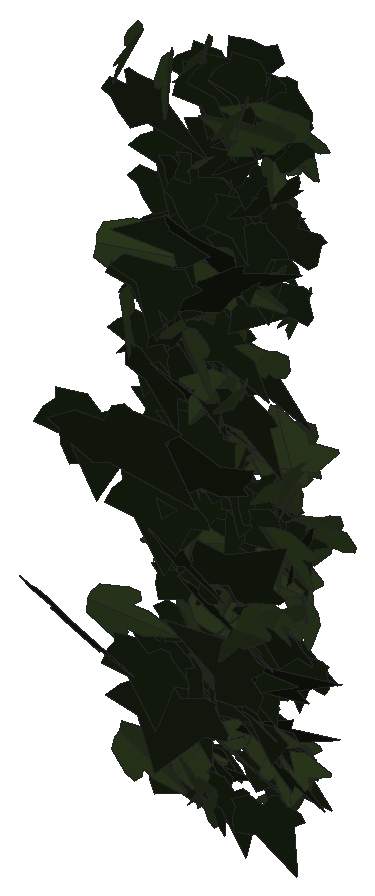
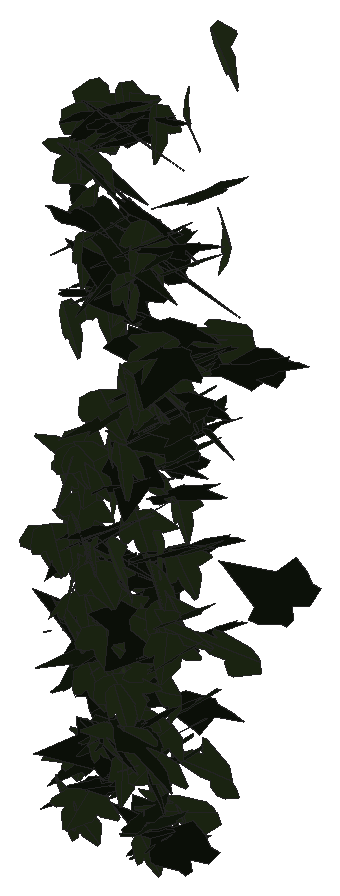
# SketchUp Ruby script. Lengths in millimetres.
U = 1.mm
M = Sketchup.active_model
def pt(a) = Geom::Point3d.new(a.map { |v| v * U })
def face(e, loops, mat)
  f = e.add_face(loops[0].map { |a| pt(a) })
  loops[1..].each { |l| e.add_face(l.map { |a| pt(a) }).erase! }
  f.material = f.back_material = mat if mat
  f
end
# faces: each face lists its corners as indices into pts; further lists are holes
def faces(e, pts, list, mat = nil) = list.each { |f| face(e, (f[0].is_a?(Array) ? f : [f]).map { |l| l.map { |i| pts[i] } }, mat) }
# xy, xz, yz: faces in a plane at the given z, y or x. An outline is a flat list of corners, or four numbers for a rectangle; further outlines are holes
def ring(l) = l.size == 4 ? [[l[0], l[1]], [l[2], l[1]], [l[2], l[3]], [l[0], l[3]]] : l.each_slice(2).to_a
def flat(e, list, mat, &to3) = list.each { |f| face(e, (f[0].is_a?(Array) ? f : [f]).map { |l| ring(l).map { |u, v| to3.(u, v) } }, mat) }
def xy(e, z, list, mat = nil) = flat(e, list, mat) { |x, y| [x, y, z] }
def xz(e, y, list, mat = nil) = flat(e, list, mat) { |x, z| [x, y, z] }
def yz(e, x, list, mat = nil) = flat(e, list, mat) { |y, z| [x, y, z] }
def lines(e, pts, list) = list.each { |a, b| e.add_line(pt(pts[a]), pt(pts[b])) }
# prism: a flat outline (further loops are holes) pulled along v
def prism(e, loops, v, mat = nil)
  f = face(e, loops, mat); d = Geom::Vector3d.new(v.map { |x| x * U })
  f.pushpull(f.normal.samedirection?(d) ? d.length : -d.length)
end
def box(e, o, s, mat = nil) = prism(e, [[o, [o[0] + s[0], o[1], o[2]], [o[0] + s[0], o[1] + s[1], o[2]], [o[0], o[1] + s[1], o[2]]]], [0, 0, s[2]], mat)
def at(x, y, z, deg = 0) = Geom::Transformation.translation(pt([x, y, z])) * Geom::Transformation.rotation(ORIGIN, Z_AXIS, deg.degrees)
def axes(o, x, y, z) = Geom::Transformation.new([*x, 0, *y, 0, *z, 0, *pt(o).to_a, 1])
def part(name) = M.definitions.add(name)
# library, detail: a bought-in or finely detailed component or shape, given as its bounding box
def library(name, o, s) = part(name).tap { |d| box(d.entities, o, s) }
def detail(e, o, s) = box(e.add_group.entities, o, s)
def put(e, d, t, mat = nil) = e.add_instance(d, t).tap { |i| i.material = mat if mat }
def group(e, t, mat = nil) = e.add_group.tap { |g| g.transformation = t; g.material = mat if mat }.entities
root = M.entities
M.materials.add("efeu1").color = [18, 25, 13]
M.materials.add("efeu2").color = [43, 57, 29]
c1 = part("ivyleaf_10")
p = [[0,12.8,-0.8],[-1.5,51.3,-10.9],[-4.9,51,-11.6],[-13.6,26.5,-7.3],[-13.2,15.9,-4.6],[-21.1,19.3,-7.2],
  [-29.5,16.3,-8.3],[-29.2,8.3,-6.2],[-19.7,-9.8,0.5],[-7.6,-13,4],[1,-12.2,5.8],[-0.4,51.1,-11.1],
  [-1.5,51.1,-10.9],[1,-12.4,5.9],[16.9,-12.4,3.5],[35.1,9.1,-5.1],[35,12.9,-6.1],[20.5,16.4,-4.9],
  [15.8,15,-3.8],[15.3,27.6,-7.1],[12.8,31.3,-7.8]]
faces(c1.entities,p,[[0,1,2,3,4,5,6,7,8,9,10],[11,12,0,13,14,15,16,17,18,19,20]],"efeu2")
c2 = part("ivyleaf_9")
p = [[39.1,54.8,31.7],[34.5,51.8,30.2],[-5.3,25.2,17.3],[-17.9,28.3,20.9],[-21.6,21.7,17],[-20.2,4.3,5.3],
  [-22.9,-0.3,2.5],[-17.1,-4,-0.6],[-2,-2.1,-1.2],[-0.7,-15.4,-10.1],[16.6,-22.3,-16.7],[21.1,-15.1,-12.5],
  [32.7,-10.7,-11],[46.1,-1.8,-6.6],[30.8,11.2,3.8]]
faces(c2.entities,p,[[0,1,2,3,4,5,6,7,8,9,10,11,12,13,14]],"efeu1")
put(root,c1,axes([1806.8,852.7,2286.1],[-0.01789,-0.27296,-1.00474],[1.7176,0.4989,-0.14398],[0.98809,-0.87218,0.23209]))
put(root,c2,axes([1814.5,923.6,2199.2],[0.8191,-0.82834,0.03911],[0.07035,-0.02486,-0.93323],[1.57668,0.43144,0.02132]))
put(root,c2,axes([1832.8,891.2,2170.1],[-0.57727,-0.84907,0.25897],[-0.09922,-0.25616,-0.90092],[1.68653,-0.30569,0.03564]))
put(root,c1,axes([1839.7,935.9,1905.6],[-0.70225,-0.77074,-0.26118],[0.21308,0.23596,-0.85451],[1.53408,-0.38559,-0.00087]))
put(root,c1,axes([1803.5,843.7,1861.3],[-0.11726,-0.14923,-0.94753],[1.74149,-0.29398,-0.0132],[-0.54765,-0.90288,0.16091]))
put(root,c2,axes([1821.7,939,1897.6],[0.48366,-0.85833,-0.13459],[-0.0231,0.13671,-0.89476],[1.65338,0.253,0.02687]))
put(root,c2,axes([1802.2,758.8,1893.8],[0.73437,-0.75336,0.79815],[0.9389,-0.63671,-0.83948],[1.86594,0.61688,0.10828]))
put(root,c1,axes([1869.4,932.1,1920.6],[-0.51931,-0.03752,0.86368],[-1.31002,-0.53851,-0.24086],[0.99542,-0.72828,0.1336]))
put(root,c2,axes([1808,939.7,1636.8],[0.25974,-0.20872,0.88748],[1.4299,-0.48258,-0.22903],[0.9829,0.75721,0.09866]))
put(root,c1,axes([1848.6,902.2,2000],[-0.29132,-0.90496,0.15875],[-0.04171,-0.15729,-0.9178],[1.74812,-0.15456,0.00456]))
put(root,c2,axes([1832.7,931.2,1936.3],[-0.41611,-0.79777,0.37994],[0.10328,-0.40278,-0.81451],[1.67854,-0.17299,0.1443]))
put(root,c2,axes([1862.1,889.3,2202],[-1.38301,0.60822,-0.28042],[0.35773,-0.21195,-0.94677],[-1.22346,-0.74951,0.04017]))
put(root,c1,axes([1814.2,907.6,1678.1],[-0.273,-0.23425,-0.87554],[1.62662,0.26004,-0.2096],[0.57405,-0.84825,0.17753]))
put(root,c2,axes([1822.8,906.1,2152.3],[0.66647,-0.8096,-0.30899],[0.01559,0.33635,-0.87198],[1.64916,0.324,0.13312]))
put(root,c2,axes([1830.3,923.7,1786.6],[0.1838,-0.89431,-0.03993],[-0.01066,0.03956,-0.89951],[1.70371,0.09673,-0.00132]))
put(root,c2,axes([1829.3,936,1822.8],[0.39894,-0.78359,-0.36918],[-0.07531,0.37077,-0.80945],[1.64684,0.20678,0.05241]))
put(root,c2,axes([1830.8,927.7,1747],[0.1742,-0.87935,0.08662],[-0.00556,-0.08739,-0.88402],[1.68167,0.0908,-0.0119]))
put(root,c2,axes([1831.3,908.6,2215.7],[0.12453,-0.93776,0.07241],[0.01529,-0.07203,-0.94004],[1.78999,0.06586,0.00299]))
put(root,c2,axes([1838.6,876.6,2258.3],[-0.41233,-0.94448,0.04012],[-0.01948,-0.03882,-0.96901],[1.79905,-0.21689,-0.00129]))
put(root,c2,axes([1821.6,922.4,2177.2],[1.26029,-0.66097,-0.01558],[0.17116,0.11189,-0.92467],[1.24661,0.65286,0.14271]))
put(root,c2,axes([1824.1,856.1,2476.1],[0.942,-0.78164,-0.39133],[0.10249,0.47612,-0.88289],[1.66049,0.41404,0.2765]))
put(root,c2,axes([1860.9,902.4,2081.1],[-1.03653,-0.55878,0.4979],[-0.58921,-0.39242,-0.77905],[1.29682,-0.62492,0.044]))
put(root,c2,axes([1844.5,913.3,2222.2],[-1.24414,-0.51874,-0.45344],[0.69635,0.26827,-0.83439],[1.1111,-0.74899,0.01519]))
put(root,c1,axes([1858.5,913.8,2251.8],[-0.93334,-0.77907,0.21994],[-0.0753,-0.23378,-0.9163],[1.53884,-0.48396,0.08856]))
put(root,c2,axes([1845.4,909.2,2009],[-0.66156,-0.74237,0.40176],[0.04025,-0.44201,-0.79845],[1.606,-0.29472,0.18551]))
put(root,c1,axes([1855.5,925.2,1937.9],[-0.4944,-0.83661,0.22386],[0.0624,-0.24305,-0.87027],[1.64707,-0.24192,0.10016]))
put(root,c2,axes([1841.6,895.6,2253.8],[-0.39531,-0.83885,0.42478],[0.05389,-0.44041,-0.85586],[1.78871,-0.17212,0.11966]))
put(root,c1,axes([1845.3,954.8,1758],[-1.57169,-0.0913,-0.2792],[0.55595,-0.1675,-0.80924],[0.05889,-0.85549,0.18825]))
put(root,c2,axes([1835.9,889.1,1806.7],[0.27514,-0.87641,-0.02007],[-0.0044,0.01996,-0.88825],[1.66842,0.14458,0.00097]))
put(root,c2,axes([1846.2,939.8,2021.7],[-0.56565,-0.83427,0.17684],[0.00413,-0.18801,-0.88333],[1.62306,-0.29027,0.06388]))
put(root,c1,axes([1852.2,942.5,2000.7],[1.14004,-0.66904,-0.05326],[0.09654,0.11631,-0.89059],[1.27368,0.59002,0.11517]))
put(root,c2,axes([1835.6,925.9,1649.3],[0.00834,-0.65503,-0.56743],[0.38392,0.55262,-0.63638],[1.60407,-0.12886,0.15526]))
put(root,c2,axes([1860.4,931.7,1708.9],[0.26844,-0.01041,0.9238],[0.22641,0.92693,-0.00772],[-1.74366,0.11876,0.14122]))
put(root,c1,axes([1846.9,933.7,1788.2],[-1.35772,0.34867,-0.38991],[0.53967,-0.2963,-0.78378],[-0.83652,-0.75707,0.12719]))
put(root,c1,axes([1841.4,925.2,1833.9],[-0.59717,0.42234,-0.76207],[0.64996,-0.68555,-0.52054],[-1.52553,-0.45741,0.07653]))
put(root,c2,axes([1841.3,910.6,2241.2],[-0.10118,-0.92287,0.20804],[0.19908,-0.21282,-0.91736],[1.78944,-0.0285,0.11382]))
put(root,c1,axes([1872.2,908.9,2007.1],[0.01108,0.13355,0.92122],[-1.01136,0.75685,-0.10636],[-1.45455,-0.52523,0.08097]))
put(root,c2,axes([1874.1,951.6,1785.5],[-0.35049,0.84553,-0.17008],[-0.02305,-0.17643,-0.864],[-1.64129,-0.17808,0.04845]))
put(root,c1,axes([1864.9,945.8,1640.5],[-0.1963,-0.82055,0.20963],[0.03786,-0.21347,-0.82578],[1.61138,-0.09494,0.04494]))
put(root,c1,axes([1824.4,854.4,1700.3],[0.46764,-0.08568,1.02242],[1.90404,-0.21322,-0.2583],[0.43319,1.02969,0.03159]))
put(root,c2,axes([1847.5,919.9,1884.8],[0.07257,-0.77738,-0.44687],[0.04508,0.44799,-0.77731],[1.70594,0.02123,0.03955]))
put(root,c2,axes([1851.2,952.4,1665.1],[-0.36095,-0.74936,0.37902],[0.20819,-0.4073,-0.75053],[1.58461,-0.11718,0.18494]))
put(root,c1,axes([1867.7,878.4,2059.1],[0.0512,-0.92071,-0.14302],[0.00898,0.14321,-0.92106],[1.7733,0.02586,0.00879]))
put(root,c2,axes([1856.7,866.6,1999.7],[-0.5786,-1.01642,-0.05268],[0.02879,0.05047,-1.06091],[1.93683,-0.30439,0.00003]))
put(root,c2,axes([1864.5,872.8,2265.3],[-0.93301,-0.83607,0.06848],[-0.03714,-0.06793,-0.96904],[1.59611,-0.49031,0.01748]))
put(root,c2,axes([1867.2,910.9,2271.7],[1.45835,0.46985,-0.32593],[-0.68222,-0.02992,-0.88587],[-0.84793,0.83216,0.15218]))
put(root,c2,axes([1852.8,939.7,1639.3],[0.20806,-0.80647,0.18433],[0.01718,-0.18476,-0.8137],[1.57436,0.1086,-0.01548]))
put(root,c1,axes([1861.4,912.4,2243.7],[0.91052,0.61423,0.55019],[0.04971,0.62447,-0.71988],[-1.56862,0.37633,0.29655]))
put(root,c1,axes([1864.4,904.9,1948.4],[0.95994,-0.72281,0.29148],[0.37879,-0.21623,-0.8806],[1.43411,0.54093,0.03748]))
put(root,c2,axes([1853,855.6,2157],[0.21213,-0.86515,0.39633],[0.1705,-0.38773,-0.87156],[1.80306,0.13845,0.03579]))
put(root,c2,axes([1857.6,911.6,1746.1],[0.16751,-0.88571,0.109],[-0.01064,-0.11007,-0.88992],[1.69836,0.08667,-0.01633]))
put(root,c2,axes([1858.4,924.5,1737.8],[0.3685,-0.73156,-0.43374],[-0.12768,0.43031,-0.75573],[1.61358,0.20112,0.03925]))
put(root,c2,axes([1871.8,896.3,2399.3],[-0.96395,-0.83413,0.08884],[0.06677,-0.12475,-0.97129],[1.5951,-0.49886,0.09434]))
put(root,c1,axes([1859.2,903.9,1662.9],[1.38379,-0.50813,-0.25575],[0.40988,-0.13827,0.88699],[-1.00207,-0.75825,0.00964]))
put(root,c2,axes([1874.8,903.8,2303.4],[-1.41791,-0.52187,-0.30455],[0.46975,0.17847,-0.9096],[1.04966,-0.78482,-0.00433]))
put(root,c2,axes([1858.9,919.6,2182.6],[0.18909,-0.92979,0.03741],[0.00496,-0.03734,-0.93509],[1.77101,0.09938,-0.00137]))
put(root,c2,axes([1851,871.6,2374.8],[0.75081,-0.79386,-0.42932],[0.13424,0.49423,-0.84907],[1.7124,0.30933,0.2548]))
put(root,c2,axes([1872.4,902.6,2000.8],[-0.74198,-0.8427,0.09054],[-0.01062,-0.09711,-0.92783],[1.61303,-0.38828,0.03554]))
put(root,c1,axes([1881.9,913.2,1651.8],[0.10191,-0.84845,-0.27109],[-0.02669,0.27074,-0.85013],[1.69498,0.05528,0.00291]))
put(root,c2,axes([1862.8,946.5,1668.6],[0.04989,-0.6379,0.56107],[0.16969,-0.55617,-0.6365],[1.60791,0.07849,0.04976]))
put(root,c1,axes([1880.8,893.9,2169],[1.06253,-0.75308,-0.07967],[-0.03732,0.08458,-0.93681],[1.44077,0.55756,0.03449]))
put(root,c1,axes([1885.4,886.7,2205.9],[-0.5776,-0.88514,-0.09861],[0.07053,0.09153,-0.93571],[1.69355,-0.3057,0.00534]))
put(root,c1,axes([1891.4,918.1,1785.4],[0.93329,-0.52338,-0.51154],[-0.32519,0.51686,-0.69263],[1.35436,0.48477,0.1862]))
put(root,c1,axes([1872.6,904.3,2276.5],[0.30526,0.69781,0.63691],[0.28094,0.61958,-0.716],[-1.77601,0.21795,-0.00379]))
put(root,c1,axes([1886.2,914,1910.4],[0.90698,-0.74407,-0.15768],[-0.03077,0.17612,-0.87996],[1.44723,0.47005,0.08011]))
put(root,c1,axes([1878,924.7,1859.6],[0.13178,-0.66748,0.6504],[0.0676,0.65361,0.66699],[-1.77241,-0.0247,0.07379]))
put(root,c1,axes([1889.3,954.5,1733.7],[-0.30036,-0.79398,-0.29062],[0.14336,0.28126,-0.80931],[1.60274,-0.17395,0.01793]))
put(root,c1,axes([1878.4,947.1,1772.5],[0.12807,-0.75129,-0.46612],[0.23676,-0.45478,0.75096],[-1.66596,-0.12238,0.07089]))
put(root,c1,axes([1883.2,962.3,1784.5],[1.36872,0.48149,-0.00307],[-0.05022,0.03389,-0.86441],[-0.91502,0.71838,0.04284]))
put(root,c2,axes([1880.4,925.2,1907.3],[1.35934,0.53164,0.03839],[0.04816,0.03029,-0.89033],[-1.0133,0.71463,0.00918]))
put(root,c1,axes([1895.3,954.9,1825.2],[-0.27382,-0.86299,-0.03822],[-0.02058,0.04054,-0.87473],[1.64393,-0.14323,-0.01732]))
put(root,c2,axes([1867.5,855.4,1959.7],[1.17753,-0.66751,-0.06586],[-0.03108,0.07458,-0.90933],[1.27619,0.61772,0.03862]))
put(root,c2,axes([1875.6,926.8,1732.7],[0.71952,-0.64055,-0.45637],[-0.23132,0.45269,-0.73607],[1.47888,0.38245,0.10691]))
put(root,c1,axes([1901.7,949.6,1835.3],[-1.01758,-0.62299,0.31586],[-0.19701,-0.32271,-0.81173],[1.31468,-0.53056,0.12284]))
put(root,c2,axes([1872.4,937.9,1735],[0.41059,-0.75981,-0.367],[0.17047,0.39729,-0.76985],[1.59684,0.15295,0.17655]))
put(root,c2,axes([1885.8,728.3,2165.2],[-0.83885,-1.03489,-0.11415],[0.08186,0.10575,-1.12484],[1.97986,-0.44285,-0.00185]))
put(root,c2,axes([1895.6,847.1,1778.6],[-1.64175,-0.51536,-0.33613],[0.54808,0.17335,-1.00485],[1.03483,-0.90942,-0.00106]))
put(root,c2,axes([1927.8,843.4,2342.1],[-1.41714,0.53945,0.32451],[-0.60835,0.10905,-0.91471],[-1.03219,-0.8049,0.09357]))
put(root,c1,axes([1901.3,909.7,2032.5],[-0.62919,-0.85871,0.06277],[-0.05364,-0.05641,-0.92013],[1.63777,-0.33174,-0.00602]))
put(root,c2,axes([1894.9,926.4,1891.4],[-0.40521,-0.48592,0.71831],[-0.41652,-0.6856,-0.52866],[1.5971,-0.30209,0.04437]))
put(root,c2,axes([1886.7,806.3,1846.7],[-0.29874,-0.9643,0.02792],[-0.00778,-0.02762,-0.97699],[1.83601,-0.15702,0.0004]))
put(root,c1,axes([1901.9,761.6,2602.5],[0.55134,-1.07798,0.08466],[0.04371,-0.08149,-1.11623],[2.05746,0.2906,0.00103]))
put(root,c2,axes([1864,870,2135.7],[1.40694,-0.58942,0.40228],[0.61842,-0.23766,-0.94534],[1.20919,0.80736,0.01541]))
put(root,c1,axes([1929.9,898,2100.2],[-1.08969,-0.14106,0.73762],[-1.34568,-0.2113,-0.58925],[0.48162,-0.90953,0.02249]))
put(root,c2,axes([1880.2,877.2,2386],[0.60878,-0.93261,0.02621],[0.01524,-0.02496,-0.98594],[1.77557,0.31997,-0.00052]))
put(root,c1,axes([1889.4,834.4,2536.5],[0.69469,-0.60969,0.76872],[0.91079,-0.60538,-0.70737],[1.63014,0.59806,0.06763]))
put(root,c1,axes([1911.1,862.6,2543.5],[-0.04605,-0.91499,-0.42909],[0.14707,0.42628,-0.91336],[1.91775,-0.05466,0.05974]))
put(root,c2,axes([1890.3,875.8,2164.5],[0.38364,-0.93513,0.04936],[0.01619,-0.04866,-0.95661],[1.78214,0.20175,-0.00194]))
put(root,c2,axes([1913.3,907.8,2108.2],[1.35362,0.0971,-0.62296],[-1.19576,0.0309,-0.7125],[-0.1,0.94497,0.08731]))
put(root,c1,axes([1908.6,890.3,2404],[-0.63553,-0.85286,-0.36926],[0.36929,0.31975,-0.91397],[1.7298,-0.38161,0.05945]))
put(root,c2,axes([1934.1,886.9,2428.5],[-1.7922,0.27966,-0.00731],[0.01218,-0.00414,-0.98232],[-0.53228,-0.9417,0.00214]))
put(root,c1,axes([1911.6,926.7,2124.5],[1.15172,-0.59939,-0.36822],[-0.04415,0.46845,-0.80067],[1.3381,0.53136,0.29052]))
put(root,c1,axes([1909.1,919.7,2219.4],[1.20101,-0.68924,-0.10856],[0.10493,0.19517,-0.91865],[1.32377,0.60985,0.17131]))
put(root,c2,axes([1930.2,869.8,2090.6],[-1.47393,-0.42705,0.3107],[-0.44203,-0.21986,-0.88113],[0.90269,-0.80496,0.07584]))
put(root,c2,axes([1898.3,899,2039.3],[0.78763,-0.65445,-0.53289],[-0.27628,0.52947,-0.76298],[1.5823,0.41822,0.13204]))
put(root,c1,axes([1899.4,862.5,2195.5],[-0.58604,0.42784,-0.84012],[0.64319,-0.77497,-0.51853],[-1.67507,-0.44725,0.09482]))
put(root,c2,axes([1904.2,890.2,2390],[-0.04068,-0.98061,-0.09477],[0.00284,0.09476,-0.98084],[1.87498,-0.02142,-0.00057]))
put(root,c2,axes([1913.6,960.9,1766.6],[-1.15944,-0.01807,-0.6065],[1.14699,-0.11783,-0.60184],[-0.13411,-0.85152,0.09615]))
put(root,c2,axes([1913.8,920.4,2082.7],[-0.68625,-0.84483,0.10318],[-0.00566,-0.11081,-0.91767],[1.61982,-0.35831,0.04051]))
put(root,c1,axes([1926.4,939.6,1885.8],[-1.2954,-0.54724,0.07313],[-0.09389,-0.05533,-0.87327],[1.04656,-0.68232,0.01217]))
put(root,c1,axes([1926.2,901.4,2337.7],[-0.37889,-0.94887,0.03635],[0.01157,-0.03841,-0.96944],[1.80719,-0.19869,0.01383]))
put(root,c1,axes([1923.8,929.7,1994],[0.46561,-0.8658,0.02358],[0.01261,-0.02264,-0.8997],[1.64836,0.24474,0.00022]))
put(root,c1,axes([1922.8,908,1908],[0.02467,-0.80066,0.39776],[0.24992,-0.39178,-0.79291],[1.68304,0.06991,0.11191]))
put(root,c1,axes([1927.6,918.6,1859.3],[-0.22995,-0.88019,-0.12853],[0.07446,0.12433,-0.88818],[1.6913,-0.12514,0.02163]))
put(root,c2,axes([1906.7,893.6,2203.9],[0.46274,-0.84332,-0.39837],[-0.03696,0.40702,-0.87347],[1.77468,0.22837,0.08568]))
put(root,c1,axes([1930.7,866.2,2158.9],[-0.46652,-0.73679,0.54659],[0.05635,-0.57182,-0.75753],[1.74508,-0.1785,0.17058]))
put(root,c1,axes([1924.6,903.9,2325.5],[-1.17544,0.74402,-0.02898],[0.02685,-0.02596,-0.96694],[-1.41684,-0.61774,0.00572]))
put(root,c1,axes([1917.1,899,1854.5],[1.44578,0.48087,-0.2889],[0.44472,0.17089,0.89887],[0.97063,-0.79457,0.01848]))
put(root,c1,axes([1913.2,862.3,1664.1],[-1.1095,0.44962,0.68947],[1.05612,-0.40933,0.73613],[1.15703,0.80477,-0.01078]))
put(root,c2,axes([1907.3,856,2387.4],[0.76207,-0.75278,-0.57248],[-0.12059,0.59893,-0.83188],[1.79588,0.35966,0.18707]))
put(root,c2,axes([1951.4,897.2,2380.2],[-1.04691,0.75007,-0.30003],[0.01212,-0.35894,-0.90903],[-1.53746,-0.51358,0.19713]))
put(root,c2,axes([1898,873.3,1896.9],[1.28684,-0.75593,0.20134],[0.28143,-0.13782,-1.01404],[1.462,0.69189,0.01798]))
put(root,c2,axes([1899.7,899.3,1784.8],[0.79092,-0.67224,0.50939],[0.56736,-0.41414,-0.78975],[1.50162,0.51055,0.03009]))
put(root,c1,axes([1941,899.4,2079.1],[-0.80715,0.60088,0.59974],[-0.65287,0.49196,-0.73547],[-1.47799,-0.54546,-0.00265]))
put(root,c2,axes([1916.2,925.8,1763.3],[0.33196,-0.9103,-0.19992],[-0.06853,0.19666,-0.92686],[1.77245,0.1781,0.00161]))
put(root,c1,axes([1915.4,922.5,1834],[0.26733,-0.48894,-0.7946],[0.59987,-0.73145,0.5058],[-1.67126,-0.34075,0.05444]))
put(root,c1,axes([1942,941,1964.9],[-0.72994,-0.75266,0.2885],[-0.09899,-0.29572,-0.84064],[1.53089,-0.378,0.0832]))
put(root,c1,axes([1934,939.7,1751.1],[-0.27778,-0.73088,0.51134],[0.30113,-0.53114,-0.71401],[1.67072,-0.02579,0.21371]))
put(root,c1,axes([1951.8,882.5,2293.1],[-0.83062,0.5177,0.7093],[-0.96358,0.49883,-0.6756],[-1.36552,-0.6669,0.04528]))
put(root,c1,axes([1930.7,974.6,1684.5],[-1.11531,-0.53911,-0.26307],[0.54009,0.07486,-0.78557],[1.00585,-0.63798,0.13012]))
put(root,c2,axes([1941.6,823.8,2061.1],[1.25814,0.19822,0.71645],[-1.3776,-0.04672,0.6808],[0.32222,-0.97372,0.11318]))
put(root,c2,axes([1907.8,899.1,2320.9],[1.36797,0.62064,-0.17745],[0.26892,0.10786,0.94959],[1.19873,-0.73245,-0.01053]))
put(root,c1,axes([1944,942.7,1831.8],[-0.72274,-0.78041,0.18899],[-0.01002,-0.20663,-0.86385],[1.52818,-0.37044,0.08372]))
put(root,c2,axes([1910.1,710.2,2172.2],[-0.42072,-0.48104,-1.08794],[1.07849,0.93036,-0.5265],[1.99056,-0.60574,0.05532]))
put(root,c2,axes([1933.1,923.6,2018.4],[-0.55388,-0.80059,0.32103],[-0.07188,-0.32666,-0.84886],[1.64004,-0.28469,0.07122]))
put(root,c1,axes([1925.5,721.7,2310.2],[-0.25563,0.38401,-1.0691],[0.40786,-1.04865,-0.40359],[-2.12316,-0.24768,0.05119]))
put(root,c2,axes([1928.7,922,1812.6],[-0.17106,-0.83891,-0.33722],[0.02335,0.33772,-0.84342],[1.72062,-0.08799,-0.02208]))
put(root,c2,axes([1939.7,873.2,2529.4],[-0.95185,-0.85702,0.03239],[-0.02632,-0.02943,-0.99227],[1.63202,-0.50032,0.00289]))
put(root,c1,axes([1950.6,911.7,2176.5],[-1.11517,-0.66588,0.30897],[-0.1504,-0.33582,-0.8736],[1.38897,-0.57098,0.15347]))
put(root,c2,axes([1940,966.4,1686.4],[-0.682,-0.76013,0.12156],[-0.04856,-0.12228,-0.83987],[1.46425,-0.3581,0.02877]))
put(root,c2,axes([1933.1,890.6,1663.1],[0.0156,-0.84083,0.22261],[-0.02162,-0.22271,-0.84077],[1.65526,0.00502,-0.01308]))
put(root,c2,axes([1939.2,893,2361.7],[-0.46534,-0.93887,0.09298],[-0.01202,-0.09442,-0.97003],[1.79556,-0.24395,0.0176]))
put(root,c2,axes([1925.9,902.5,2337.8],[0.78454,-0.80483,-0.35202],[-0.00547,0.38761,-0.88958],[1.67185,0.37895,0.16228]))
put(root,c1,axes([1954.4,903.9,2304.6],[-0.62359,-0.8956,-0.12697],[0.02808,0.12974,-0.95316],[1.72131,-0.32657,-0.03045]))
put(root,c2,axes([1980.5,884.6,2535.2],[-1.6661,0.45236,0.16553],[-0.39515,-0.04451,-0.97638],[-0.82724,-0.88982,0.133]))
put(root,c2,axes([1944.5,901.4,2352],[1.04329,-0.2604,-0.75335],[-0.99312,0.57391,-0.57807],[1.14674,0.73393,0.18475]))
put(root,c2,axes([1940.2,861.3,2520.9],[-0.38618,-0.97376,-0.16203],[0.04775,0.16028,-0.99465],[1.87814,-0.2043,-0.00803]))
put(root,c2,axes([1932.8,936.2,1747.3],[0.37149,-0.80873,0.27072],[0.14479,-0.2601,-0.83186],[1.61665,0.20913,0.01229]))
put(root,c2,axes([1940.1,920.9,2016.5],[-0.13046,-0.82223,-0.38597],[0.01234,0.38661,-0.82476],[1.72866,-0.06481,-0.02324]))
put(root,c2,axes([1987.8,901.1,1974.2],[-1.07605,0.45589,0.56706],[-0.98896,0.24966,-0.71882],[-0.96928,-0.76084,0.1039]))
put(root,c2,axes([1931.6,915.6,2168.2],[0.97223,-0.80431,-0.34052],[-0.15384,0.34925,-0.94621],[1.65516,0.50491,0.11207]))
put(root,c2,axes([1936.3,942.4,1688.4],[0.3887,-0.55464,-0.62506],[0.09582,0.65046,-0.56073],[1.58754,0.09654,0.18689]))
put(root,c1,axes([1934.4,918.2,1725.6],[1.48471,0.12833,0.4222],[0.78655,0.08811,-0.7904],[-0.29438,0.88265,0.01752]))
put(root,c1,axes([1959.7,950.1,1643.2],[-0.26322,-0.75555,0.39257],[0.01503,-0.39884,-0.76482],[1.6204,-0.11903,0.07086]))
put(root,c2,axes([1937.4,838.6,2321.6],[-0.70329,-0.23006,0.96265],[0.90938,-0.94135,-0.04155],[1.64966,0.42084,0.43331]))
put(root,c1,axes([1974.1,909.4,2075.6],[1.29543,0.26824,-0.58825],[-1.14946,-0.04096,-0.71752],[-0.43906,0.8987,0.14287]))
put(root,c2,axes([1974.2,889.9,1924.8],[-1.64452,-0.35779,0.20506],[0.42028,0.00062,0.93163],[-0.66284,0.88808,0.08196]))
put(root,c2,axes([1933.7,918.5,1722],[0.99007,0.2606,0.68132],[1.12142,0.3432,-0.58116],[-0.81842,0.78551,0.02789]))
put(root,c1,axes([1972.7,913.6,1978.4],[0.10759,-0.12748,-0.93577],[-0.47816,0.90163,-0.138],[1.73263,0.25674,0.02002]))
put(root,c2,axes([1947.2,929.1,1744.5],[-0.31328,-0.73641,0.45049],[0.19582,-0.47207,-0.7341],[1.63127,-0.08476,0.17464]))
put(root,c1,axes([1954.7,889.9,2109.7],[0.20739,-0.7675,0.5544],[0.46942,-0.51578,-0.76252],[1.73973,0.23066,0.13966]))
put(root,c1,axes([1969.5,913.4,2097.1],[-1.18002,-0.70202,0.08547],[-0.10686,-0.06445,-0.93662],[1.34171,-0.62256,0.00058]))
put(root,c2,axes([1954.7,880.1,2505.8],[-0.63488,-0.91813,0.23362],[-0.02991,-0.24228,-0.97461],[1.80281,-0.32735,0.0661]))
put(root,c1,axes([1964.9,856.3,2163.3],[0.20554,-0.95409,0.09059],[0.02658,-0.08959,-0.96018],[1.8238,0.10883,0.00378]))
put(root,c2,axes([1940.2,887.6,1712.3],[0.0215,-0.55256,0.69409],[0.77207,-0.61411,-0.49549],[1.50161,0.32366,0.24482]))
put(root,c2,axes([1948,866.3,1928.5],[-0.84385,0.12379,0.79146],[1.3943,-0.30329,0.45785],[0.61677,0.855,0.04782]))
put(root,c2,axes([1949,920.8,2006],[0.36659,-0.84865,-0.26493],[0.07678,0.27914,-0.86484],[1.69028,0.17138,0.09674]))
put(root,c1,axes([1971.8,964.4,1679.7],[0.81867,-0.67352,-0.26046],[-0.14415,0.25942,-0.79591],[1.36678,0.43078,0.07207]))
put(root,c2,axes([1961.6,871.2,2527.2],[-0.64656,-0.94987,-0.04401],[0.02343,0.04234,-1.00879],[1.80957,-0.33994,-0.00267]))
put(root,c1,axes([1953.6,900.4,1886.3],[-1.32539,0.29604,-0.53495],[0.85547,-0.30174,-0.75213],[-0.78878,-0.82468,0.08316]))
put(root,c1,axes([1978.4,921.4,2077.6],[-1.62762,0.38411,0.00997],[-0.20658,-0.21816,-0.90534],[-0.70149,-0.82697,0.24346]))
put(root,c1,axes([1969.4,932.2,1964.4],[-0.51668,0.82044,-0.30303],[0.0072,-0.31619,-0.85946],[-1.66455,-0.25604,0.09034]))
put(root,c1,axes([1976.2,932.4,2019.1],[0.57614,-0.86255,-0.00942],[-0.00062,0.00987,-0.91413],[1.64171,0.30271,0.00296]))
put(root,c1,axes([1981.8,920.7,2099.6],[-0.97743,-0.7449,0.21719],[-0.07971,-0.23346,-0.89975],[1.47458,-0.50638,0.09533]))
put(root,c2,axes([1952.6,928.5,1855.4],[1.01365,-0.64442,-0.27208],[-0.02717,0.33188,-0.81402],[1.33102,0.49754,0.19058]))
put(root,c2,axes([1959.5,880.2,2512.8],[-0.06447,-0.96377,0.45458],[-0.00301,-0.45476,-0.96428],[2.02805,-0.03131,0.01302]))
put(root,c1,axes([1944.7,899,1928.2],[0.02855,-0.36595,-0.87914],[1.45005,-0.52283,0.23064],[-1.08718,-0.70694,0.28452]))
put(root,c2,axes([1965.6,883.8,2324.5],[-0.3376,-0.95115,-0.13532],[0.05655,0.13211,-0.96754],[1.82759,-0.17979,0.00494]))
put(root,c2,axes([1958.3,891.8,2396.5],[0.87609,-0.70377,-0.5022],[-0.17401,0.52613,-0.82111],[1.63625,0.43277,0.18157]))
put(root,c2,axes([1963.9,915.9,1711.2],[1.20188,-0.51188,-0.38719],[-0.50194,0.28825,-0.81123],[1.11362,0.68237,0.05223]))
put(root,c1,axes([1978.9,917.5,2032.8],[-0.65146,-0.77182,-0.36409],[0.30687,0.32673,-0.84421],[1.59492,-0.37812,0.01371]))
put(root,c2,axes([1961,870.2,2143.3],[0.46075,-0.91626,-0.03594],[-0.0171,0.0348,-0.9477],[1.74508,0.24226,0.0002]))
put(root,c2,axes([2002.5,861.1,2399.8],[-0.18488,0.9131,0.32755],[-0.42614,0.29919,-0.90045],[-1.79638,-0.16495,0.1799]))
put(root,c2,axes([1967.5,942.8,1816.9],[-0.02891,-0.77389,0.42218],[0.03605,-0.42243,-0.77367],[1.67739,-0.00426,0.0239]))
put(root,c2,axes([2000.1,827.8,1853.5],[-0.31083,-1.08391,-0.06907],[0.02666,-0.07194,1.09587],[-2.06692,0.16207,0.02452]))
put(root,c1,axes([1986.5,897.5,1962.4],[0.85773,-0.75495,-0.23389],[-0.14218,0.22735,-0.87778],[1.49746,0.45402,0.05063]))
put(root,c2,axes([1970.6,853.8,2359.4],[-1.18294,-0.40287,-0.62601],[1.27205,0.05712,-0.70038],[0.6239,-0.88031,0.24104]))
put(root,c2,axes([2000.1,885.1,2470.7],[-1.47352,0.41184,-0.4684],[0.50225,-0.46021,-0.84084],[-1.07556,-0.77913,0.24907]))
put(root,c1,axes([1989.3,899.1,1892.1],[-0.73831,-0.82469,-0.05564],[0.02493,0.05532,-0.91131],[1.57293,-0.38798,-0.01167]))
put(root,c2,axes([1973.8,870,2369.9],[-0.35102,-0.95277,-0.0685],[0.02528,0.0672,-0.97045],[1.81781,-0.18492,0.00027]))
put(root,c1,axes([1944.4,840.8,2309.6],[0.13177,-0.03854,1.09488],[2.08469,0.02307,-0.06845],[-0.03921,1.09682,0.03991]))
put(root,c2,axes([1973.1,890.9,1660.3],[0.00735,-0.78759,-0.37309],[-0.04497,0.37286,-0.78735],[1.658,0.0136,-0.0197]))
put(root,c2,axes([2016,890.1,2468],[-1.58955,0.49732,0.17445],[-0.32535,0.05358,-0.9712],[-0.94881,-0.85154,0.04077]))
put(root,c1,axes([1981.6,919.4,1704.6],[0.86931,0.73847,-0.0626],[-0.07251,-0.05004,-0.86829],[-1.40864,0.45831,0.00606]))
put(root,c1,axes([1986.4,928.8,2081.2],[0.16863,-0.64485,-0.65367],[0.26759,0.65849,-0.63054],[1.72693,-0.03907,0.16153]))
put(root,c1,axes([1990.3,899.3,2363.9],[-0.14715,-0.91247,-0.32673],[0.19566,0.3182,-0.91297],[1.83418,-0.10715,0.07118]))
put(root,c1,axes([1987,937.6,1919.2],[-0.15809,0.85943,-0.28009],[-0.05106,-0.28349,-0.86191],[-1.71959,-0.0706,0.05135]))
put(root,c2,axes([1998.1,882.6,2292.8],[-1.30487,-0.64324,0.22955],[-0.11754,-0.26554,-0.92855],[1.29451,-0.6725,0.14708]))
put(root,c1,axes([1986.5,890.4,2436.8],[0.11223,0.89388,-0.41727],[-0.05756,-0.41618,-0.89582],[-1.87657,0.06622,0.00253]))
put(root,c1,axes([1985.8,909.2,1954.4],[-0.38183,-0.60862,0.64247],[0.58538,-0.66565,-0.53453],[1.57928,0.09959,0.35347]))
put(root,c1,axes([1996.7,817.5,2522.2],[0.02329,-0.98949,-0.23253],[0.07752,0.23284,-0.98866],[1.93295,0.00259,0.04245]))
put(root,c2,axes([1982.7,912.1,1989.2],[-0.1931,-0.87954,-0.25125],[0.01155,0.25213,-0.8851],[1.74086,-0.09924,-0.022]))
put(root,c2,axes([1988.9,877.5,2531.2],[-0.68047,-1.00167,0.1176],[-0.03796,-0.11773,-1.06337],[1.9191,-0.3575,0.02067]))
put(root,c2,axes([1981.7,897.3,1870.9],[-0.49525,-0.64301,0.58185],[0.43098,-0.63679,-0.60245],[1.59317,-0.02762,0.34385]))
put(root,c2,axes([1980.6,786.6,2321.7],[0.12781,0.70227,-0.87889],[-0.14767,0.88125,0.69822],[2.13601,0.0189,0.10086]))
put(root,c1,axes([1993.7,823.7,1908.4],[-0.29496,-0.64223,-0.88155],[0.46313,0.8476,-0.66028],[2.02346,-0.28762,0.02262]))
put(root,c1,axes([2005.3,922.2,1883.8],[0.9403,-0.67286,-0.31123],[-0.38876,0.23599,-0.83444],[1.35634,0.53411,-0.0234]))
put(root,c1,axes([2000.2,896.8,2084.2],[1.63537,0.41996,0.12321],[-0.21488,-0.04959,0.9564],[0.80477,-0.86665,0.00498]))
put(root,c2,axes([1961.6,869.2,1823.7],[1.61313,0.43122,-0.43161],[0.72582,0.20222,0.95095],[0.90636,-0.92941,0.00665]))
put(root,c1,axes([2006.6,935.3,1989.8],[-0.83352,-0.78933,0.05645],[-0.04526,-0.05136,-0.90268],[1.5054,-0.43858,0.00412]))
put(root,c1,axes([2005.2,861.1,2312.3],[-0.19884,-0.95509,0.05949],[-0.00936,-0.05931,-0.96079],[1.82123,-0.10458,0.00156]))
put(root,c2,axes([2008.1,888.1,2495.4],[-0.3436,-0.25589,0.9416],[-0.98641,-0.78618,-0.31303],[1.57341,-0.54875,0.00938]))
put(root,c1,axes([2029.4,828.5,2498.5],[-0.85871,-0.04257,-0.89484],[-1.49279,-0.4653,0.41762],[-0.82375,0.88759,0.17601]))
put(root,c1,axes([2010.3,930.1,1983.5],[-1.55918,-0.34443,0.10191],[-0.15236,-0.07234,-0.888],[0.66643,-0.82238,0.03542]))
put(root,c1,axes([1990.8,889.1,1985.5],[-1.42419,0.31004,-0.44507],[0.71178,-0.25436,-0.80599],[-0.74771,-0.83268,0.08049]))
put(root,c2,axes([2011.8,898.1,1965.3],[0.01065,0.26119,-0.90162],[-1.09232,0.71442,0.2034],[1.41368,0.55005,0.16395]))
put(root,c1,axes([2017.6,856.1,2507.8],[-1.34208,-0.59037,0.36839],[-0.28358,-0.38422,-0.90094],[1.29368,-0.69668,0.18469]))
put(root,c1,axes([2011.1,904.7,2068.7],[0.07543,-0.89494,0.25146],[-0.04026,-0.2525,-0.89527],[1.76875,0.03242,-0.0311]))
put(root,c1,axes([1996.8,890.2,2472.5],[-1.68672,0.22484,-0.37665],[0.65699,-0.16642,-0.9116],[-0.51512,-0.94848,0.07067]))
put(root,c2,axes([2011.9,901.1,1848.4],[-1.12654,-0.5599,0.38395],[-0.13304,-0.45642,-0.77335],[1.28521,-0.53802,0.25649]))
put(root,c2,axes([2028.8,869.2,2375.6],[-1.83199,-0.14515,0.08264],[-0.15708,-0.00689,-0.97345],[0.27636,-0.9661,-0.00547]))
put(root,c1,axes([2010.1,868.8,2489.8],[-0.38919,-0.87716,-0.45135],[0.22478,0.43586,-0.90057],[1.86394,-0.23571,0.01436]))
put(root,c1,axes([2012.6,903.1,2265.3],[0.13803,-0.94381,-0.07882],[0.00758,0.07935,-0.94654],[1.8025,0.07194,0.01002]))
